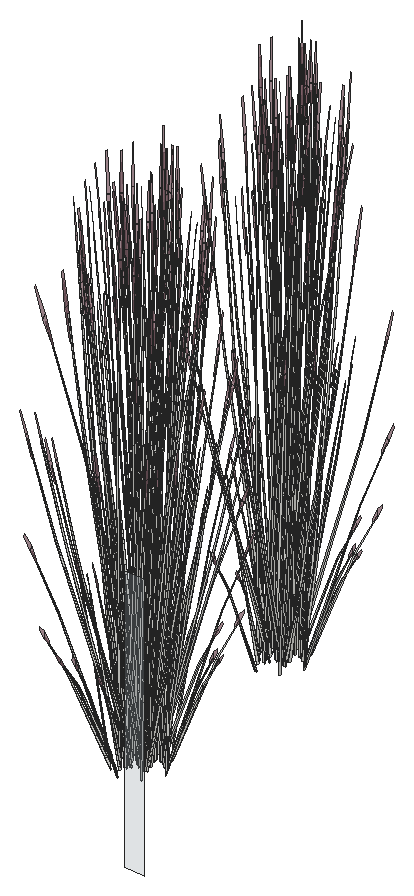
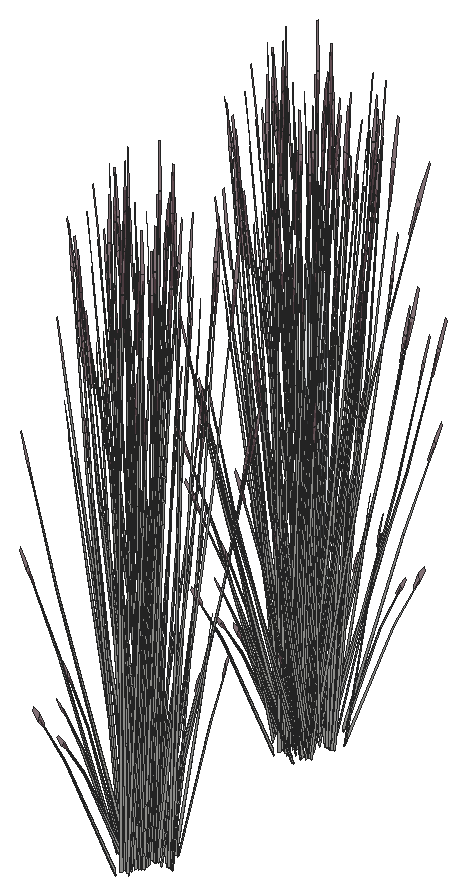
# SketchUp Ruby script. Lengths in inches.
U = 1.inch
M = Sketchup.active_model
def pt(a) = Geom::Point3d.new(a.map { |v| v * U })
def face(e, loops, mat)
  f = e.add_face(loops[0].map { |a| pt(a) })
  loops[1..].each { |l| e.add_face(l.map { |a| pt(a) }).erase! }
  f.material = f.back_material = mat if mat
  f
end
# faces: each face lists its corners as indices into pts; further lists are holes
def faces(e, pts, list, mat = nil) = list.each { |f| face(e, (f[0].is_a?(Array) ? f : [f]).map { |l| l.map { |i| pts[i] } }, mat) }
# xy, xz, yz: faces in a plane at the given z, y or x. An outline is a flat list of corners, or four numbers for a rectangle; further outlines are holes
def ring(l) = l.size == 4 ? [[l[0], l[1]], [l[2], l[1]], [l[2], l[3]], [l[0], l[3]]] : l.each_slice(2).to_a
def flat(e, list, mat, &to3) = list.each { |f| face(e, (f[0].is_a?(Array) ? f : [f]).map { |l| ring(l).map { |u, v| to3.(u, v) } }, mat) }
def xy(e, z, list, mat = nil) = flat(e, list, mat) { |x, y| [x, y, z] }
def xz(e, y, list, mat = nil) = flat(e, list, mat) { |x, z| [x, y, z] }
def yz(e, x, list, mat = nil) = flat(e, list, mat) { |y, z| [x, y, z] }
def lines(e, pts, list) = list.each { |a, b| e.add_line(pt(pts[a]), pt(pts[b])) }
# prism: a flat outline (further loops are holes) pulled along v
def prism(e, loops, v, mat = nil)
  f = face(e, loops, mat); d = Geom::Vector3d.new(v.map { |x| x * U })
  f.pushpull(f.normal.samedirection?(d) ? d.length : -d.length)
end
def box(e, o, s, mat = nil) = prism(e, [[o, [o[0] + s[0], o[1], o[2]], [o[0] + s[0], o[1] + s[1], o[2]], [o[0], o[1] + s[1], o[2]]]], [0, 0, s[2]], mat)
def at(x, y, z, deg = 0) = Geom::Transformation.translation(pt([x, y, z])) * Geom::Transformation.rotation(ORIGIN, Z_AXIS, deg.degrees)
def axes(o, x, y, z) = Geom::Transformation.new([*x, 0, *y, 0, *z, 0, *pt(o).to_a, 1])
def part(name) = M.definitions.add(name)
# library, detail: a bought-in or finely detailed component or shape, given as its bounding box
def library(name, o, s) = part(name).tap { |d| box(d.entities, o, s) }
def detail(e, o, s) = box(e.add_group.entities, o, s)
def put(e, d, t, mat = nil) = e.add_instance(d, t).tap { |i| i.material = mat if mat }
def group(e, t, mat = nil) = e.add_group.tap { |g| g.transformation = t; g.material = mat if mat }.entities
root = M.entities
M.materials.add("Glass_Basic_01").color = [161, 173, 186]
M.materials["Glass_Basic_01"].alpha = 0.25
M.materials.add("LightPink_Translucent").color = [144, 107, 117]
M.materials["LightPink_Translucent"].alpha = 0.75
c1 = part("blade")
p = [[2.15,0.21,22],[0,0.17,0],[0.09,0.45,0],[2.18,0.31,22],[2.29,0.31,22],[0.38,0.45,0],
  [2.48,0.24,33],[2.49,0.24,33],[2.48,0.22,33]]
faces(c1.entities,p,[[0,1,2,3],[4,5,2,3],[6,3,4,7],[8,0,3,6]])
c2 = part("seeds")
p = [[0.3,-0.1,1.38],[-0.01,-0.03,1.59],[-0.01,-0.03,0.03],[0.14,-0.07,-0.07],[0.29,-0.03,3],[0.15,0.01,3.11]]
faces(c2.entities,p,[[0,1,2,3],[1,0,4,5]],"LightPink_Translucent")
c3 = part("blade with seeds")
put(c3.entities,c1,at(0,0,0))
put(c3.entities,c2,axes([2.4,0.25,30.99],[1.5799,-0.05474,1.17369],[-0.12525,1.92788,0.29478],[-0.07173,-0.02425,1.56792]))
xz(root,180,[[312,149,314,175]],"Glass_Basic_01")
put(root,c3,axes([302.88,192.37,149.1875],[-0.11649,0.09547,1.20808],[-0.34886,-0.1671,-0.25981],[0.06467,-0.20781,0.51652]))
put(root,c3,axes([302.35,192.7,151.21],[-0.19559,-0.38351,-0.60019],[0.40262,-0.21373,0.07243],[-0.04574,-0.1853,0.84903]))
put(root,c3,axes([301.08,192.1875,149.1875],[-0.02482,0.15429,1.20808],[-0.36278,0.12916,-0.25981],[-0.0848,-0.19943,0.51652]))
put(root,c3,axes([302.02,191.85,148.26],[-0.06874,0.01699,1.48974],[-0.38012,-0.19128,-0.22758],[0.00638,-0.15955,0.25375]))
put(root,c3,axes([303.17,193.07,151.21],[0.01066,-0.43628,-0.60019],[0.44902,0.0293,0.07243],[0.04739,-0.18483,0.84903]))
put(root,c3,axes([302.21,192.62,150.95],[-0.40284,-0.11824,-0.43168],[0.13808,-0.40538,-0.33437],[-0.03694,-0.16321,0.82598]))
put(root,c3,axes([302.46,191.61,149.34],[0.05257,0.27504,0.97034],[-0.29163,-0.15233,0.71294],[0.03138,-0.14083,0.21373]))
put(root,c3,axes([303.08,192.93,150.95],[-0.29336,-0.31691,-0.43168],[0.3099,-0.27755,-0.33437],[0.04464,-0.16102,0.82598]))
put(root,c3,axes([300.96,191.9375,149.34],[0.21377,0.16416,0.97034],[-0.31132,0.09868,0.71294],[-0.06661,-0.12616,0.21373]))
put(root,c3,axes([301.47,192.81,151.21],[-0.34944,-0.22798,-0.60019],[0.24834,-0.39949,0.07243],[-0.1266,-0.13612,0.84903]))
put(root,c3,axes([300.79,192.43,148.26],[-0.0397,0.06213,1.48974],[-0.40116,0.13396,-0.22758],[-0.09691,-0.12186,0.25375]))
put(root,c3,axes([301.45,194.14,148.77],[-0.1683,-0.48366,-0.58997],[0.48479,-0.17419,-0.15484],[-0.0186,-0.16378,1.30225]))
put(root,c3,axes([303.7,192.66,148.26],[-0.06134,-0.03716,1.48974],[-0.15755,-0.41512,-0.22758],[0.10629,-0.11265,0.25375]))
put(root,c3,axes([301.31,192.82,150.95],[-0.40438,0.11212,-0.43168],[-0.07074,-0.4246,-0.33437],[-0.10862,-0.12168,0.82598]))
put(root,c3,axes([303.7,193.83,151.21],[0.21406,-0.37215,-0.60019],[0.37511,0.26448,0.07243],[0.12781,-0.13483,0.84903]))
put(root,c3,axes([301.38,192.75,149],[-0.25622,-0.47263,0],[0.42866,-0.26357,-0.43598],[0.09763,-0.06003,1.38303]))
put(root,c3,axes([303.6875,193.66,150.95],[-0.10528,-0.43067,-0.43168],[0.39868,-0.07534,-0.33437],[0.11425,-0.11568,0.82598]))
put(root,c3,axes([301.95,192.18,148.8],[-0.28319,0.27058,-0.03288],[-0.25948,-0.29635,-0.1491],[-0.01827,-0.08397,0.4918]))
put(root,c3,axes([302.31,195.39,149.81],[0.35414,0.19019,1.27785],[-0.34693,0.40974,0.50532],[-0.1554,-0.24285,1.07126]))
put(root,c3,axes([300.46,194.07,148.7],[0,-0.47166,-0.41945],[0.45849,0,0],[0,-0.10742,1.33059]))
put(root,c3,axes([301.73,192.68,148.7],[0.38354,-0.23583,-0.41945],[0.22925,0.42288,0],[0.08735,-0.05371,1.33059]))
put(root,c3,axes([304.01,193.49,149.1875],[-0.1464,-0.01397,1.20808],[-0.14998,-0.37477,-0.25981],[0.17985,-0.10602,0.51652]))
put(root,c3,axes([302.19,193.64,148.74],[0.27603,-0.35451,-0.52676],[0.34289,0.32147,-0.13825],[0.11061,-0.08844,1.16273]))
put(root,c3,axes([304.18,192.8,149.34],[-0.1365,0.2401,0.97034],[-0.11733,-0.32258,0.71294],[0.11274,-0.08083,0.21373]))
put(root,c3,axes([301.7,194.26,148.87],[0.19883,-0.425,-0.37796],[0.41314,0.20454,0.1819],[0,-0.09797,1.2135]))
put(root,c3,axes([301.89,194.05,149.25],[-0.04775,-0.53819,-0.2458],[0.49736,-0.03254,-0.42242],[0.08758,-0.07169,1.34921]))
put(root,c3,axes([300.65,194.08,148.71],[0.28606,-0.29428,-0.2617],[0.28606,0.29428,0.2617],[0,-0.09479,1.17405]))
put(root,c3,axes([300.54,192.67,148.8],[-0.11822,0.38513,-0.03288],[-0.36385,-0.11847,-0.1491],[-0.05524,-0.06299,0.4918]))
put(root,c3,axes([301.66,194.62,149.25],[-0.46151,-0.22505,-0.2458],[0.22222,-0.475,-0.42242],[-0.0145,-0.11662,1.34921]))
put(root,c3,axes([300.34,194.43,149],[-0.51243,0,0],[0,-0.52715,-0.43598],[0,-0.12006,1.38303]))
put(root,c3,axes([301.82,192.86,148.71],[0.38233,0.1167,-0.2617],[-0.09626,0.41098,0.2617],[0.07708,-0.04739,1.17405]))
put(root,c3,axes([300.74,194.29,148.97],[-0.38118,0.39654,0.25983],[-0.38142,-0.39237,-0.30828],[-0.01331,-0.11261,1.39295]))
put(root,c3,axes([301.95,194.48,149.06],[0.46174,0.2286,0.2033],[-0.22222,0.475,0.42242],[0,-0.1095,1.35626]))
put(root,c3,axes([301.77,195.12,149.06],[0.10862,-0.55889,-0.19793],[0.515,0.09742,0.43313],[-0.08999,-0.07718,1.32161]))
put(root,c3,axes([301.8,194.16,149.3],[-0.44501,0.02912,0.37796],[-0.04024,-0.48332,-0.1819],[0.07967,-0.04899,1.2135]))
put(root,c3,axes([300.65,194.51,149.09],[0,0.47166,0.41945],[-0.45849,0,0],[0,-0.10742,1.33059]))
put(root,c3,axes([303.87,194.62,150.95],[0.11102,-0.42903,-0.43168],[0.38064,0.14706,-0.33437],[0.15325,-0.03934,0.82598]))
put(root,c3,axes([303.27,192.87,149.01],[0.25622,-0.47263,0],[0.42866,0.26357,-0.43598],[0.09763,0.06003,1.38303]))
put(root,c3,axes([301.74,194.89,148.87],[-0.24618,-0.39589,-0.37796],[0.37289,-0.27878,0.1819],[-0.07967,-0.04899,1.2135]))
put(root,c3,axes([301.79,194.33,148.99],[0.17817,0.52741,0.38653],[-0.50909,0.1834,0.15168],[0.00622,-0.09691,1.34202]))
put(root,c3,axes([304.28,194.74,148.67],[-0.26394,0.0566,1.1961],[-0.04201,-0.45055,0.06846],[0.18486,-0.06819,0.68062]))
put(root,c3,axes([304.76,194.34,148.91],[-0.25407,-0.3016,-0.05481],[0.27826,-0.27635,-0.2485],[0.07884,-0.01946,0.81966]))
put(root,c3,axes([301.7,194.75,149.3],[-0.19883,0.425,0.37796],[-0.41314,-0.20454,-0.1819],[0,-0.09797,1.2135]))
put(root,c3,axes([302.43,194.375,148.86],[0,-0.54574,0],[0.51243,0,0],[0,0,1.51605]))
put(root,c3,axes([303.05,193.12,149.09],[-0.38354,-0.23583,0.41945],[0.22925,-0.42288,0],[0.08735,0.05371,1.33059]))
put(root,c3,axes([303.8,194.77,151.21],[0.3601,-0.20831,-0.60019],[0.20068,0.4288,0.07243],[0.17399,-0.04871,0.84903]))
put(root,c3,axes([301.51,195.04,148.74],[-0.42629,-0.07733,-0.52676],[0.08996,-0.47699,-0.13825],[-0.12722,-0.0578,1.16273]))
put(root,c3,axes([302.18,194.03,148.99],[-0.33979,0.42804,0.38653],[-0.40368,-0.37784,0.15168],[0.08192,-0.04272,1.34202]))
put(root,c3,axes([302.56,194.8,148.94],[-0.38118,-0.40596,-0.0518],[0.38142,-0.40621,0],[-0.01331,-0.01418,1.48322]))
put(root,c3,axes([301.59,193.33,149.09],[-0.11838,0.46875,0.14904],[-0.43321,-0.13265,0.29641],[0.07483,-0.00228,1.35512]))
put(root,c3,axes([301.42,193.71,148.35],[-0.40337,0.18883,1.08919],[-0.12839,-0.54182,0.42321],[0.24769,0.00901,1.23883]))
put(root,c3,axes([302.5,193.85,149.21],[0.07906,-0.42093,0.12232],[0.38625,0.07307,-0.3493],[0.07029,0.04322,1.07074]))
put(root,c3,axes([301.83,194.85,148.99],[0.51796,0.09937,0.38653],[-0.10541,0.56124,0.15168],[-0.07569,-0.05419,1.34202]))
put(root,c3,axes([304.57,194.44,148.26],[-0.02142,-0.07161,1.48974],[0.14855,-0.41887,-0.22758],[0.14984,-0.00603,0.25375]))
put(root,c3,axes([302.33,193.96,149.3],[-0.24618,-0.39589,0.37796],[0.37289,-0.27878,-0.1819],[0.07967,0.04899,1.2135]))
put(root,c3,axes([301.0625,195.77,148.71],[-0.09626,-0.41098,-0.2617],[0.38233,-0.1167,0.2617],[-0.07708,-0.04739,1.17405]))
put(root,c3,axes([301.55,195.74,149.09],[0.44036,-0.12519,0.14904],[0.10874,0.46588,0.29641],[-0.03927,-0.06788,1.35512]))
put(root,c3,axes([302.46,193.99,149.25],[0.41376,-0.31314,-0.2458],[0.27514,0.44246,-0.42242],[0.10209,0.04493,1.34921]))
put(root,c3,axes([300.96,195.95,148.7],[-0.38354,-0.23583,-0.41945],[0.22925,-0.42288,0],[-0.08735,-0.05371,1.33059]))
put(root,c3,axes([303.5,193.15,148.7],[0.38354,0.23583,-0.41945],[-0.22925,0.42288,0],[0.08735,0.05371,1.33059]))
put(root,c3,axes([302.78,194.5,148.86],[0.45849,0,0],[0,0.4883,0],[0,0,1.50718]))
put(root,c3,axes([302,195.11,149.25],[-0.41376,0.31314,-0.2458],[-0.27514,-0.44246,-0.42242],[-0.10209,-0.04493,1.34921]))
put(root,c3,axes([302.91,193.35,149.09],[-0.44036,0.12519,0.14904],[-0.10874,-0.46588,0.29641],[0.03927,0.06788,1.35512]))
put(root,c3,axes([303.4,193.33,148.71],[0.09626,0.41098,-0.2617],[-0.38233,0.1167,0.2617],[0.07708,0.04739,1.17405]))
put(root,c3,axes([302.63,194.25,149.01],[-0.51796,-0.09937,0.41563],[0.10541,-0.56124,0.1631],[0.07569,0.05419,1.44303]))
put(root,c3,axes([302.21,195.64,148.86],[-0.13371,-0.40664,0],[0.38182,-0.1424,0],[0,0,1.30413]))
put(root,c3,axes([301.96,195.25,149.21],[-0.07906,0.42093,0.12232],[-0.38625,-0.07307,-0.3493],[-0.07029,-0.04322,1.07074]))
put(root,c3,axes([302.71,195.58,148.85],[0.43024,-0.16003,-0.16218],[0.15118,0.46099,0.00007],[0.04749,-0.01769,1.46908]))
put(root,c3,axes([302.86,195.77,149.09],[0.11838,-0.46875,0.14904],[0.43321,0.13265,0.29641],[-0.07483,0.00228,1.35512]))
put(root,c3,axes([302.77,194.71,148.87],[0.28606,0.30466,0],[-0.28606,0.30466,0],[0,0,1.42996]))
put(root,c3,axes([303.54,194.57,149.09],[-0.32198,-0.34356,0.14904],[0.32447,-0.33323,0.29641],[-0.03556,0.07016,1.35512]))
put(root,c3,axes([302.94,194.06,148.74],[0.42629,0.07733,-0.52676],[-0.08996,0.47699,-0.13825],[0.12722,0.0578,1.16273]))
put(root,c3,axes([304.83,194.89,149.34],[-0.2532,0.07787,0.97034],[0.11918,-0.32181,0.71294],[0.13432,0.02202,0.21373]))
put(root,c3,axes([302.12,195.82,148.86],[-0.41314,-0.21175,0],[0.19883,-0.43999,0],[0,0,1.37455]))
put(root,c3,axes([302.46,195.26,149.08],[-0.40016,-0.37963,-0.21282],[0.33672,-0.42629,0.46574],[-0.10776,0.04441,1.42109]))
put(root,c3,axes([301.41,195.98,149.09],[0.38354,0.23583,0.41945],[-0.22925,0.42288,0],[-0.08735,-0.05371,1.33059]))
put(root,c3,axes([302.76,194.35,149.3],[0.19883,-0.425,0.37796],[0.41314,0.20454,-0.1819],[0,0.09797,1.2135]))
put(root,c3,axes([302.68,194.59,148.9375],[0,0.54548,-0.04762],[-0.51243,0,0],[0,0.01714,1.5153]))
put(root,c3,axes([302.72,194.21,148.87],[0.24618,0.39589,-0.37796],[-0.37289,0.27878,0.1819],[0.07967,0.04899,1.2135]))
put(root,c3,axes([301.1875,196.23,149],[-0.25622,0.47263,0],[-0.42866,-0.26357,-0.43598],[-0.09763,-0.06003,1.38303]))
put(root,c3,axes([303.8,194.59,149.09],[0,-0.47166,0.41945],[0.45849,0,0],[0,0.10742,1.33059]))
put(root,c3,axes([302.66,194.94,149.3],[0.44501,-0.02912,0.37796],[0.04024,0.48332,-0.1819],[-0.07967,0.04899,1.2135]))
put(root,c3,axes([302.93,194.45,149.21],[0.38182,-0.13755,0.12232],[0.13371,0.39278,-0.3493],[0,0.08644,1.07074]))
put(root,c3,axes([302.26,195.17,148.87],[-0.44501,0.02912,-0.37796],[-0.04024,-0.48332,0.1819],[-0.07967,0.04899,1.2135]))
put(root,c3,axes([304.35,195.41,149.1875],[-0.0987,-0.116,1.20808],[0.12841,-0.38374,-0.25981],[0.19968,0.05198,0.51652]))
put(root,c3,axes([302.59,195.83,148.86],[0.41314,0.21175,0],[-0.19883,0.43999,0],[0,0,1.47801]))
put(root,c3,axes([302.75,196.3,148.85],[-0.25302,-0.47428,-0.04344],[0.42866,-0.26357,0.43598],[-0.10563,0.04516,1.38235]))
put(root,c3,axes([302.66,195.15,149.21],[0.30276,0.28338,0.12232],[-0.25254,0.31972,-0.3493],[-0.07029,0.04322,1.07074]))
put(root,c3,axes([303.45,195.64,151.21],[0.40965,0.01136,-0.60019],[-0.02751,0.47821,0.07243],[0.17355,0.05047,0.84903]))
put(root,c3,axes([302.99,196.02,149.09],[0.38354,-0.23583,0.41945],[0.22925,0.42288,0],[-0.08735,0.05371,1.33059]))
put(root,c3,axes([302.44,195.65,148.9375],[0.17817,0.54185,-0.05079],[-0.50909,0.18987,0],[0.00622,0.01892,1.45452]))
put(root,c3,axes([302.64,196.24,148.71],[-0.38233,-0.1167,-0.2617],[0.09626,-0.41098,0.2617],[-0.07708,0.04739,1.17405]))
put(root,c3,axes([304.12,194.67,149.01],[0.51243,0,0],[0,0.52715,-0.43598],[0,0.12006,1.38303]))
put(root,c3,axes([303.91,194.9375,148.86],[-0.51218,-0.00377,-0.04204],[0,-0.52715,0.42192],[-0.0161,0.12,1.33776]))
put(root,c3,axes([302.8,194.48,149.25],[0.46151,0.22505,-0.2458],[-0.22222,0.475,-0.42242],[0.0145,0.11662,1.34921]))
put(root,c3,axes([303.8,195.02,148.71],[-0.28606,0.29428,-0.2617],[-0.28606,-0.29428,0.2617],[0,0.09479,1.17405]))
put(root,c3,axes([302.57,195.04,149.25],[0.04775,0.53819,-0.2458],[-0.49736,0.03254,-0.42242],[-0.08758,0.07169,1.34921]))
put(root,c3,axes([302.75,194.83,148.87],[-0.19883,0.425,-0.37796],[-0.41314,-0.20454,0.1819],[0,0.09797,1.2135]))
put(root,c3,axes([302.27,195.45,148.74],[-0.27603,0.35451,-0.52676],[-0.34289,-0.32147,-0.13825],[-0.11061,0.08844,1.16273]))
put(root,c3,axes([302.76,196.05,148.97],[0.51304,0.1533,0.25983],[-0.12835,0.54797,-0.30828],[-0.08491,0.06858,1.39295]))
put(root,c3,axes([302.73,196.42,148.7],[-0.38354,0.23583,-0.41945],[-0.22925,-0.42288,0],[-0.08735,0.05371,1.33059]))
put(root,c3,axes([304,195.03,148.7],[0,0.47166,-0.41945],[-0.45849,0,0],[0,0.10742,1.33059]))
put(root,c3,axes([303.42,196,149.34],[-0.23074,-0.13562,0.97034],[0.29794,-0.1378,0.71294],[0.08036,0.11673,0.21373]))
put(root,c3,axes([300.52,195.35,150.95],[0.10528,0.43067,-0.43168],[-0.39868,0.07534,-0.33437],[-0.11425,0.11568,0.82598]))
put(root,c3,axes([303.08,196.35,149],[0.25622,0.47263,0],[-0.42866,0.26357,-0.43598],[-0.09763,0.06003,1.38303]))
put(root,c3,axes([303.48,196.51,148.26],[0.02986,-0.06809,1.48974],[0.37589,-0.20055,-0.22758],[0.11396,0.1038,0.25375]))
put(root,c3,axes([302.86,194.48,149.4],[-0.01119,-0.44408,1.19347],[0.50665,0.11511,0.50532],[-0.11983,0.243,1.12654]))
put(root,c3,axes([302.99,194.96,148.77],[0.15027,0.43184,-0.5847],[-0.43285,0.15553,-0.15346],[0.01661,0.14623,1.29063]))
put(root,c3,axes([302.9,196.19,150.95],[0.40438,-0.11212,-0.43168],[0.07074,0.4246,-0.33437],[0.10862,0.12168,0.82598]))
put(root,c3,axes([303.46,196.62,149.25],[-0.26279,-0.01479,0.88755],[0.17355,-0.31417,0.49003],[0.10382,0.11162,0.6962]))
put(root,c3,axes([302.6,195.86,149.1875],[0.00723,-0.15635,1.20808],[0.34559,-0.17464,-0.25981],[0.10668,0.18713,0.51652]))
put(root,c3,axes([301.03,197.16,149.34],[-0.01061,-0.28045,0.97034],[0.26501,0.20003,0.71294],[-0.05212,0.13367,0.21373]))
put(root,c3,axes([301.73,196.49,148.26],[0.06632,-0.02567,1.48974],[0.39894,0.14126,-0.22758],[0.01167,0.15921,0.25375]))
put(root,c3,axes([301.13,196.08,151.23],[0.29336,0.31691,-0.47917],[-0.3099,0.27755,-0.37115],[-0.04464,0.16102,0.91684]))
put(root,c3,axes([300.8125,196.56,149.38],[0.37228,-0.08352,0.05498],[0.08559,0.3365,-0.7291],[-0.0236,0.17034,0.65354]))
put(root,c3,axes([302,196.39,150.95],[0.40284,0.11824,-0.43168],[-0.13808,0.40538,-0.33437],[0.03694,0.16321,0.82598]))
put(root,c3,axes([301.04,195.9375,151.51],[-0.01066,0.43628,-0.66621],[-0.44902,-0.0293,0.0804],[-0.04739,0.18483,0.94242]))
put(root,c3,axes([301.85,196.3125,151.21],[0.19559,0.38351,-0.60019],[-0.40262,0.21373,0.07243],[0.04574,0.1853,0.84903]))
put(root,c3,axes([300.72,196.91,149.1875],[0.12932,-0.07441,1.20808],[0.31929,0.22435,-0.25981],[-0.09503,0.19413,0.51652]))
put(root,c3,axes([300.89,196.55,149.84],[0.009,-0.24349,1.30391],[0.40497,0.12861,0.18019],[-0.03509,0.2595,0.61571]))
put(root,c3,axes([300.88,211.78,149.1875],[-0.11649,0.09547,1.20808],[-0.34886,-0.1671,-0.25981],[0.06467,-0.20781,0.51652]))
put(root,c3,axes([300.35,212.11,151.21],[-0.19559,-0.38351,-0.60019],[0.40262,-0.21373,0.07243],[-0.04574,-0.1853,0.84903]))
put(root,c3,axes([300.02,211.26,148.26],[-0.06874,0.01699,1.48974],[-0.38012,-0.19128,-0.22758],[0.00638,-0.15955,0.25375]))
put(root,c3,axes([301.17,212.48,151.21],[0.01066,-0.43628,-0.60019],[0.44902,0.0293,0.07243],[0.04739,-0.18483,0.84903]))
put(root,c3,axes([300.21,212.03,150.95],[-0.40284,-0.11824,-0.43168],[0.13808,-0.40538,-0.33437],[-0.03694,-0.16321,0.82598]))
put(root,c3,axes([300.46,211.02,149.34],[0.05257,0.27504,0.97034],[-0.29163,-0.15233,0.71294],[0.03138,-0.14083,0.21373]))
put(root,c3,axes([301.08,212.34,150.95],[-0.29336,-0.31691,-0.43168],[0.3099,-0.27755,-0.33437],[0.04464,-0.16102,0.82598]))
put(root,c3,axes([299.45,213.55,148.77],[-0.1683,-0.48366,-0.58997],[0.48479,-0.17419,-0.15484],[-0.0186,-0.16378,1.30225]))
put(root,c3,axes([301.7,212.07,148.26],[-0.06134,-0.03716,1.48974],[-0.15755,-0.41512,-0.22758],[0.10629,-0.11265,0.25375]))
put(root,c3,axes([301.7,213.24,151.21],[0.21406,-0.37215,-0.60019],[0.37511,0.26448,0.07243],[0.12781,-0.13483,0.84903]))
put(root,c3,axes([299.38,212.16,149],[-0.25622,-0.47263,0],[0.42866,-0.26357,-0.43598],[0.09763,-0.06003,1.38303]))
put(root,c3,axes([301.6875,213.07,150.95],[-0.10528,-0.43067,-0.43168],[0.39868,-0.07534,-0.33437],[0.11425,-0.11568,0.82598]))
put(root,c3,axes([299.95,211.59,148.8],[-0.28319,0.27058,-0.03288],[-0.25948,-0.29635,-0.1491],[-0.01827,-0.08397,0.4918]))
put(root,c3,axes([298.46,213.48,148.7],[0,-0.47166,-0.41945],[0.45849,0,0],[0,-0.10742,1.33059]))
put(root,c3,axes([299.73,212.08,148.7],[0.38354,-0.23583,-0.41945],[0.22925,0.42288,0],[0.08735,-0.05371,1.33059]))
put(root,c3,axes([302.01,212.9,149.1875],[-0.1464,-0.01397,1.20808],[-0.14998,-0.37477,-0.25981],[0.17985,-0.10602,0.51652]))
put(root,c3,axes([300.19,213.05,148.74],[0.27603,-0.35451,-0.52676],[0.34289,0.32147,-0.13825],[0.11061,-0.08844,1.16273]))
put(root,c3,axes([302.18,212.21,149.34],[-0.1365,0.2401,0.97034],[-0.11733,-0.32258,0.71294],[0.11274,-0.08083,0.21373]))
put(root,c3,axes([299.7,213.67,148.87],[0.19883,-0.425,-0.37796],[0.41314,0.20454,0.1819],[0,-0.09797,1.2135]))
put(root,c3,axes([299.89,213.46,149.25],[-0.04775,-0.53819,-0.2458],[0.49736,-0.03254,-0.42242],[0.08758,-0.07169,1.34921]))
put(root,c3,axes([298.65,213.49,148.71],[0.28606,-0.29428,-0.2617],[0.28606,0.29428,0.2617],[0,-0.09479,1.17405]))
put(root,c3,axes([299.66,214.03,149.25],[-0.46151,-0.22505,-0.2458],[0.22222,-0.475,-0.42242],[-0.0145,-0.11662,1.34921]))
put(root,c3,axes([299.82,212.27,148.71],[0.38233,0.1167,-0.2617],[-0.09626,0.41098,0.2617],[0.07708,-0.04739,1.17405]))
put(root,c3,axes([299.95,213.88,149.06],[0.46174,0.2286,0.2033],[-0.22222,0.475,0.42242],[0,-0.1095,1.35626]))
put(root,c3,axes([299.8,213.57,149.3],[-0.44501,0.02912,0.37796],[-0.04024,-0.48332,-0.1819],[0.07967,-0.04899,1.2135]))
put(root,c3,axes([298.65,213.92,149.09],[0,0.47166,0.41945],[-0.45849,0,0],[0,-0.10742,1.33059]))
put(root,c3,axes([301.87,214.02,150.95],[0.11102,-0.42903,-0.43168],[0.38064,0.14706,-0.33437],[0.15325,-0.03934,0.82598]))
put(root,c3,axes([301.27,212.28,149.01],[0.25622,-0.47263,0],[0.42866,0.26357,-0.43598],[0.09763,0.06003,1.38303]))
put(root,c3,axes([299.79,213.74,148.99],[0.17817,0.52741,0.38653],[-0.50909,0.1834,0.15168],[0.00622,-0.09691,1.34202]))
put(root,c3,axes([302.28,214.14,148.67],[-0.26394,0.0566,1.1961],[-0.04201,-0.45055,0.06846],[0.18486,-0.06819,0.68062]))
put(root,c3,axes([302.76,213.75,148.91],[-0.25407,-0.3016,-0.05481],[0.27826,-0.27635,-0.2485],[0.07884,-0.01946,0.81966]))
put(root,c3,axes([299.7,214.16,149.3],[-0.19883,0.425,0.37796],[-0.41314,-0.20454,-0.1819],[0,-0.09797,1.2135]))
put(root,c3,axes([300.43,213.78,148.86],[0,-0.54574,0],[0.51243,0,0],[0,0,1.51605]))
put(root,c3,axes([301.05,212.52,149.09],[-0.38354,-0.23583,0.41945],[0.22925,-0.42288,0],[0.08735,0.05371,1.33059]))
put(root,c3,axes([301.8,214.18,151.21],[0.3601,-0.20831,-0.60019],[0.20068,0.4288,0.07243],[0.17399,-0.04871,0.84903]))
put(root,c3,axes([300.18,213.44,148.99],[-0.33979,0.42804,0.38653],[-0.40368,-0.37784,0.15168],[0.08192,-0.04272,1.34202]))
put(root,c3,axes([300.56,214.21,148.94],[-0.38118,-0.40596,-0.0518],[0.38142,-0.40621,0],[-0.01331,-0.01418,1.48322]))
put(root,c3,axes([299.59,212.74,149.09],[-0.11838,0.46875,0.14904],[-0.43321,-0.13265,0.29641],[0.07483,-0.00228,1.35512]))
put(root,c3,axes([299.42,213.11,148.35],[-0.40337,0.18883,1.08919],[-0.12839,-0.54182,0.42321],[0.24769,0.00901,1.23883]))
put(root,c3,axes([300.5,213.26,149.21],[0.07906,-0.42093,0.12232],[0.38625,0.07307,-0.3493],[0.07029,0.04322,1.07074]))
put(root,c3,axes([299.83,214.26,148.99],[0.51796,0.09937,0.38653],[-0.10541,0.56124,0.15168],[-0.07569,-0.05419,1.34202]))
put(root,c3,axes([302.57,213.85,148.26],[-0.02142,-0.07161,1.48974],[0.14855,-0.41887,-0.22758],[0.14984,-0.00603,0.25375]))
put(root,c3,axes([300.33,213.37,149.3],[-0.24618,-0.39589,0.37796],[0.37289,-0.27878,-0.1819],[0.07967,0.04899,1.2135]))
put(root,c3,axes([299.55,215.15,149.09],[0.44036,-0.12519,0.14904],[0.10874,0.46588,0.29641],[-0.03927,-0.06788,1.35512]))
put(root,c3,axes([300.46,213.39,149.25],[0.41376,-0.31314,-0.2458],[0.27514,0.44246,-0.42242],[0.10209,0.04493,1.34921]))
put(root,c3,axes([301.5,212.5625,148.7],[0.38354,0.23583,-0.41945],[-0.22925,0.42288,0],[0.08735,0.05371,1.33059]))
put(root,c3,axes([300.78,213.91,148.86],[0.45849,0,0],[0,0.4883,0],[0,0,1.50718]))
put(root,c3,axes([300.91,212.76,149.09],[-0.44036,0.12519,0.14904],[-0.10874,-0.46588,0.29641],[0.03927,0.06788,1.35512]))
put(root,c3,axes([301.4,212.74,148.71],[0.09626,0.41098,-0.2617],[-0.38233,0.1167,0.2617],[0.07708,0.04739,1.17405]))
put(root,c3,axes([300.63,213.66,149.01],[-0.51796,-0.09937,0.41563],[0.10541,-0.56124,0.1631],[0.07569,0.05419,1.44303]))
put(root,c3,axes([300.21,215.04,148.86],[-0.13371,-0.40664,0],[0.38182,-0.1424,0],[0,0,1.30413]))
put(root,c3,axes([299.96,214.66,149.21],[-0.07906,0.42093,0.12232],[-0.38625,-0.07307,-0.3493],[-0.07029,-0.04322,1.07074]))
put(root,c3,axes([300.71,214.99,148.85],[0.43024,-0.16003,-0.16218],[0.15118,0.46099,0.00007],[0.04749,-0.01769,1.46908]))
put(root,c3,axes([300.86,215.18,149.09],[0.11838,-0.46875,0.14904],[0.43321,0.13265,0.29641],[-0.07483,0.00228,1.35512]))
put(root,c3,axes([300.77,214.12,148.87],[0.28606,0.30466,0],[-0.28606,0.30466,0],[0,0,1.42996]))
put(root,c3,axes([301.54,213.98,149.09],[-0.32198,-0.34356,0.14904],[0.32447,-0.33323,0.29641],[-0.03556,0.07016,1.35512]))
put(root,c3,axes([300.94,213.46,148.74],[0.42629,0.07733,-0.52676],[-0.08996,0.47699,-0.13825],[0.12722,0.0578,1.16273]))
put(root,c3,axes([302.83,214.3,149.34],[-0.2532,0.07787,0.97034],[0.11918,-0.32181,0.71294],[0.13432,0.02202,0.21373]))
put(root,c3,axes([300.12,215.23,148.86],[-0.41314,-0.21175,0],[0.19883,-0.43999,0],[0,0,1.37455]))
put(root,c3,axes([300.76,213.76,149.3],[0.19883,-0.425,0.37796],[0.41314,0.20454,-0.1819],[0,0.09797,1.2135]))
put(root,c3,axes([300.68,214,148.9375],[0,0.54548,-0.04762],[-0.51243,0,0],[0,0.01714,1.5153]))
put(root,c3,axes([300.72,213.62,148.87],[0.24618,0.39589,-0.37796],[-0.37289,0.27878,0.1819],[0.07967,0.04899,1.2135]))
put(root,c3,axes([301.8,214,149.09],[0,-0.47166,0.41945],[0.45849,0,0],[0,0.10742,1.33059]))
put(root,c3,axes([300.66,214.35,149.3],[0.44501,-0.02912,0.37796],[0.04024,0.48332,-0.1819],[-0.07967,0.04899,1.2135]))
put(root,c3,axes([300.93,213.86,149.21],[0.38182,-0.13755,0.12232],[0.13371,0.39278,-0.3493],[0,0.08644,1.07074]))
put(root,c3,axes([302.35,214.8125,149.1875],[-0.0987,-0.116,1.20808],[0.12841,-0.38374,-0.25981],[0.19968,0.05198,0.51652]))
put(root,c3,axes([300.59,215.24,148.86],[0.41314,0.21175,0],[-0.19883,0.43999,0],[0,0,1.47801]))
put(root,c3,axes([300.75,215.7,148.85],[-0.25302,-0.47428,-0.04344],[0.42866,-0.26357,0.43598],[-0.10563,0.04516,1.38235]))
put(root,c3,axes([300.66,214.56,149.21],[0.30276,0.28338,0.12232],[-0.25254,0.31972,-0.3493],[-0.07029,0.04322,1.07074]))
put(root,c3,axes([301.45,215.05,151.21],[0.40965,0.01136,-0.60019],[-0.02751,0.47821,0.07243],[0.17355,0.05047,0.84903]))
put(root,c3,axes([300.99,215.43,149.09],[0.38354,-0.23583,0.41945],[0.22925,0.42288,0],[-0.08735,0.05371,1.33059]))
put(root,c3,axes([300.44,215.06,148.9375],[0.17817,0.54185,-0.05079],[-0.50909,0.18987,0],[0.00622,0.01892,1.45452]))
put(root,c3,axes([300.64,215.64,148.71],[-0.38233,-0.1167,-0.2617],[0.09626,-0.41098,0.2617],[-0.07708,0.04739,1.17405]))
put(root,c3,axes([302.12,214.08,149.01],[0.51243,0,0],[0,0.52715,-0.43598],[0,0.12006,1.38303]))
put(root,c3,axes([301.91,214.35,148.86],[-0.51218,-0.00377,-0.04204],[0,-0.52715,0.42192],[-0.0161,0.12,1.33776]))
put(root,c3,axes([300.8,213.89,149.25],[0.46151,0.22505,-0.2458],[-0.22222,0.475,-0.42242],[0.0145,0.11662,1.34921]))
put(root,c3,axes([301.8,214.42,148.71],[-0.28606,0.29428,-0.2617],[-0.28606,-0.29428,0.2617],[0,0.09479,1.17405]))
put(root,c3,axes([300.57,214.45,149.25],[0.04775,0.53819,-0.2458],[-0.49736,0.03254,-0.42242],[-0.08758,0.07169,1.34921]))
put(root,c3,axes([300.75,214.24,148.87],[-0.19883,0.425,-0.37796],[-0.41314,-0.20454,0.1819],[0,0.09797,1.2135]))
put(root,c3,axes([300.76,215.46,148.97],[0.51304,0.1533,0.25983],[-0.12835,0.54797,-0.30828],[-0.08491,0.06858,1.39295]))
put(root,c3,axes([300.73,215.83,148.7],[-0.38354,0.23583,-0.41945],[-0.22925,-0.42288,0],[-0.08735,0.05371,1.33059]))
put(root,c3,axes([302,214.43,148.7],[0,0.47166,-0.41945],[-0.45849,0,0],[0,0.10742,1.33059]))
put(root,c3,axes([301.42,215.41,149.34],[-0.23074,-0.13562,0.97034],[0.29794,-0.1378,0.71294],[0.08036,0.11673,0.21373]))
put(root,c3,axes([301.08,215.76,149],[0.25622,0.47263,0],[-0.42866,0.26357,-0.43598],[-0.09763,0.06003,1.38303]))
put(root,c3,axes([301.48,215.92,148.26],[0.02986,-0.06809,1.48974],[0.37589,-0.20055,-0.22758],[0.11396,0.1038,0.25375]))
